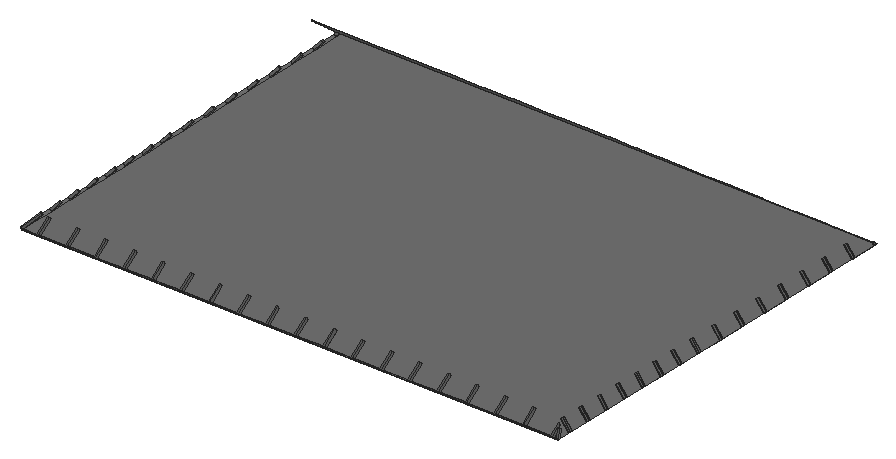
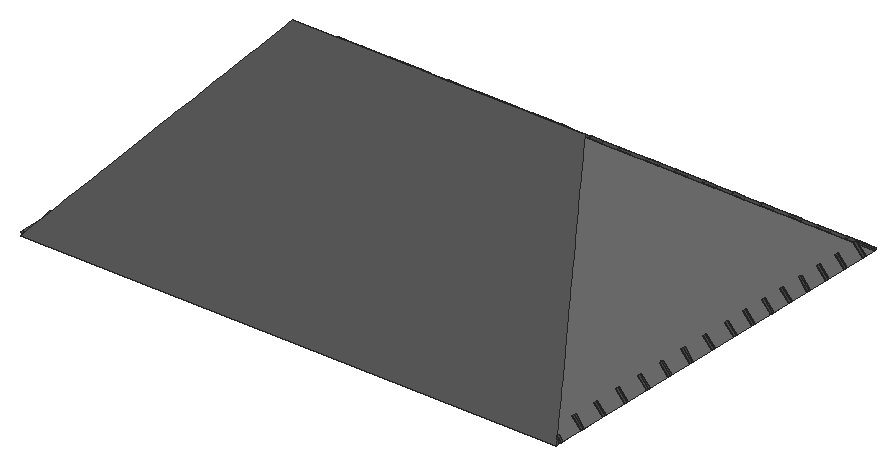
# SketchUp Ruby script. Lengths in inches.
U = 1.inch
M = Sketchup.active_model
def pt(a) = Geom::Point3d.new(a.map { |v| v * U })
def face(e, loops, mat)
  f = e.add_face(loops[0].map { |a| pt(a) })
  loops[1..].each { |l| e.add_face(l.map { |a| pt(a) }).erase! }
  f.material = f.back_material = mat if mat
  f
end
# faces: each face lists its corners as indices into pts; further lists are holes
def faces(e, pts, list, mat = nil) = list.each { |f| face(e, (f[0].is_a?(Array) ? f : [f]).map { |l| l.map { |i| pts[i] } }, mat) }
# xy, xz, yz: faces in a plane at the given z, y or x. An outline is a flat list of corners, or four numbers for a rectangle; further outlines are holes
def ring(l) = l.size == 4 ? [[l[0], l[1]], [l[2], l[1]], [l[2], l[3]], [l[0], l[3]]] : l.each_slice(2).to_a
def flat(e, list, mat, &to3) = list.each { |f| face(e, (f[0].is_a?(Array) ? f : [f]).map { |l| ring(l).map { |u, v| to3.(u, v) } }, mat) }
def xy(e, z, list, mat = nil) = flat(e, list, mat) { |x, y| [x, y, z] }
def xz(e, y, list, mat = nil) = flat(e, list, mat) { |x, z| [x, y, z] }
def yz(e, x, list, mat = nil) = flat(e, list, mat) { |y, z| [x, y, z] }
def lines(e, pts, list) = list.each { |a, b| e.add_line(pt(pts[a]), pt(pts[b])) }
# prism: a flat outline (further loops are holes) pulled along v
def prism(e, loops, v, mat = nil)
  f = face(e, loops, mat); d = Geom::Vector3d.new(v.map { |x| x * U })
  f.pushpull(f.normal.samedirection?(d) ? d.length : -d.length)
end
def box(e, o, s, mat = nil) = prism(e, [[o, [o[0] + s[0], o[1], o[2]], [o[0] + s[0], o[1] + s[1], o[2]], [o[0], o[1] + s[1], o[2]]]], [0, 0, s[2]], mat)
def at(x, y, z, deg = 0) = Geom::Transformation.translation(pt([x, y, z])) * Geom::Transformation.rotation(ORIGIN, Z_AXIS, deg.degrees)
def axes(o, x, y, z) = Geom::Transformation.new([*x, 0, *y, 0, *z, 0, *pt(o).to_a, 1])
def part(name) = M.definitions.add(name)
# library, detail: a bought-in or finely detailed component or shape, given as its bounding box
def library(name, o, s) = part(name).tap { |d| box(d.entities, o, s) }
def detail(e, o, s) = box(e.add_group.entities, o, s)
def put(e, d, t, mat = nil) = e.add_instance(d, t).tap { |i| i.material = mat if mat }
def group(e, t, mat = nil) = e.add_group.tap { |g| g.transformation = t; g.material = mat if mat }.entities
root = M.entities
M.materials.add("[Color M05]").color = [114, 114, 114]
xy(root,407.09,[[338.37,286.64,788.76,621.71]],"[Color M05]")
xz(root,298,[[338.37,407.09,336.88,408.43,344.33,416.75,345.82,415.41],[788.76,407.09,782.3,415.41,783.88,416.64,790.34,408.32]],"[Color M05]")
xz(root,299.21,[[338.37,407.09,345.82,415.41,344.33,416.75,336.88,408.43],[788.76,407.09,790.34,408.32,783.88,416.64,782.3,415.41]],"[Color M05]")
xz(root,317.375,[[338.37,407.09,336.88,408.43,344.33,416.75,345.82,415.41],[788.76,407.09,782.3,415.41,783.88,416.64,790.34,408.32]],"[Color M05]")
xz(root,318.58,[[338.37,407.09,345.82,415.41,344.33,416.75,336.88,408.43],[788.76,407.09,790.34,408.32,783.88,416.64,782.3,415.41]],"[Color M05]")
xz(root,336.74,[[338.37,407.09,336.88,408.43,344.33,416.75,345.82,415.41],[788.76,407.09,782.3,415.41,783.88,416.64,790.34,408.32]],"[Color M05]")
xz(root,337.95,[[338.37,407.09,345.82,415.41,344.33,416.75,336.88,408.43],[788.76,407.09,790.34,408.32,783.88,416.64,782.3,415.41]],"[Color M05]")
xz(root,356.11,[[338.37,407.09,336.88,408.43,344.33,416.75,345.82,415.41],[788.76,407.09,782.3,415.41,783.88,416.64,790.34,408.32]],"[Color M05]")
xz(root,357.32,[[338.37,407.09,345.82,415.41,344.33,416.75,336.88,408.43],[788.76,407.09,790.34,408.32,783.88,416.64,782.3,415.41]],"[Color M05]")
xz(root,375.48,[[338.37,407.09,336.88,408.43,344.33,416.75,345.82,415.41],[788.76,407.09,782.3,415.41,783.88,416.64,790.34,408.32]],"[Color M05]")
xz(root,376.69,[[338.37,407.09,345.82,415.41,344.33,416.75,336.88,408.43],[788.76,407.09,790.34,408.32,783.88,416.64,782.3,415.41]],"[Color M05]")
xz(root,394.85,[[338.37,407.09,336.88,408.43,344.33,416.75,345.82,415.41],[788.76,407.09,782.3,415.41,783.88,416.64,790.34,408.32]],"[Color M05]")
xz(root,396.0625,[[338.37,407.09,345.82,415.41,344.33,416.75,336.88,408.43],[788.76,407.09,790.34,408.32,783.88,416.64,782.3,415.41]],"[Color M05]")
xz(root,414.22,[[338.37,407.09,336.88,408.43,344.33,416.75,345.82,415.41],[788.76,407.09,782.3,415.41,783.88,416.64,790.34,408.32]],"[Color M05]")
xz(root,415.43,[[338.37,407.09,345.82,415.41,344.33,416.75,336.88,408.43],[788.76,407.09,790.34,408.32,783.88,416.64,782.3,415.41]],"[Color M05]")
xz(root,433.3,[[338.37,407.09,336.88,408.43,344.33,416.75,345.82,415.41]],"[Color M05]")
xz(root,433.59,[[788.76,407.09,782.3,415.41,783.88,416.64,790.34,408.32]],"[Color M05]")
xz(root,434.8,[[338.37,407.09,345.82,415.41,344.33,416.75,336.88,408.43],[788.76,407.09,790.34,408.32,783.88,416.64,782.3,415.41]],"[Color M05]")
xz(root,456.21,[[338.37,407.09,336.88,408.43,344.33,416.75,345.82,415.41]],"[Color M05]")
xz(root,456.8,[[788.76,407.09,782.3,415.41,783.88,416.64,790.34,408.32]],"[Color M05]")
xz(root,457.71,[[338.37,407.09,345.82,415.41,344.33,416.75,336.88,408.43]],"[Color M05]")
xz(root,458.01,[[788.76,407.09,790.34,408.32,783.88,416.64,782.3,415.41]],"[Color M05]")
xz(root,479.13,[[338.37,407.09,336.88,408.43,344.33,416.75,345.82,415.41]],"[Color M05]")
xz(root,480.02,[[788.76,407.09,782.3,415.41,783.88,416.64,790.34,408.32]],"[Color M05]")
xz(root,480.63,[[338.37,407.09,345.82,415.41,344.33,416.75,336.88,408.43]],"[Color M05]")
xz(root,481.23,[[788.76,407.09,790.34,408.32,783.88,416.64,782.3,415.41]],"[Color M05]")
xz(root,502.04,[[338.37,407.09,336.88,408.43,344.33,416.75,345.82,415.41]],"[Color M05]")
xz(root,503.23,[[788.76,407.09,782.3,415.41,783.88,416.64,790.34,408.32]],"[Color M05]")
xz(root,503.54,[[338.37,407.09,345.82,415.41,344.33,416.75,336.88,408.43]],"[Color M05]")
xz(root,504.44,[[788.76,407.09,790.34,408.32,783.88,416.64,782.3,415.41]],"[Color M05]")
xz(root,524.95,[[338.37,407.09,336.88,408.43,344.33,416.75,345.82,415.41]],"[Color M05]")
xz(root,526.45,[[338.37,407.09,345.82,415.41,344.33,416.75,336.88,408.43],[788.76,407.09,782.3,415.41,783.88,416.64,790.34,408.32]],"[Color M05]")
xz(root,527.66,[[788.76,407.09,790.34,408.32,783.88,416.64,782.3,415.41]],"[Color M05]")
xz(root,547.87,[[338.37,407.09,336.88,408.43,344.33,416.75,345.82,415.41]],"[Color M05]")
xz(root,549.37,[[338.37,407.09,345.82,415.41,344.33,416.75,336.88,408.43]],"[Color M05]")
xz(root,549.66,[[788.76,407.09,782.3,415.41,783.88,416.64,790.34,408.32]],"[Color M05]")
xz(root,550.87,[[788.76,407.09,790.34,408.32,783.88,416.64,782.3,415.41]],"[Color M05]")
xz(root,570.78,[[338.37,407.09,336.88,408.43,344.33,416.75,345.82,415.41]],"[Color M05]")
xz(root,572.28,[[338.37,407.09,345.82,415.41,344.33,416.75,336.88,408.43]],"[Color M05]")
xz(root,572.875,[[788.76,407.09,782.3,415.41,783.88,416.64,790.34,408.32]],"[Color M05]")
xz(root,574.08,[[788.76,407.09,790.34,408.32,783.88,416.64,782.3,415.41]],"[Color M05]")
xz(root,593.69,[[338.37,407.09,336.88,408.43,344.33,416.75,345.82,415.41]],"[Color M05]")
xz(root,595.19,[[338.37,407.09,345.82,415.41,344.33,416.75,336.88,408.43]],"[Color M05]")
xz(root,596.09,[[788.76,407.09,782.3,415.41,783.88,416.64,790.34,408.32]],"[Color M05]")
xz(root,597.3,[[788.76,407.09,790.34,408.32,783.88,416.64,782.3,415.41]],"[Color M05]")
xz(root,616.61,[[338.37,407.09,336.88,408.43,340.22,412.16,341.71,410.82]],"[Color M05]")
xz(root,618.11,[[338.37,407.09,340.73,409.73,339.24,411.06,336.88,408.43]],"[Color M05]")
xz(root,619.3,[[788.76,407.09,787.4,408.85,788.98,410.08,790.34,408.32]],"[Color M05]")
yz(root,352.12,[[286.64,407.09,298,415.41,296.82,417.03,285.45,408.71]],"[Color M05]")
yz(root,353.62,[[286.64,407.09,285.45,408.71,296.82,417.03,298,415.41]],"[Color M05]")
yz(root,376.12,[[286.64,407.09,298,415.41,296.82,417.03,285.45,408.71]],"[Color M05]")
yz(root,377.62,[[286.64,407.09,285.45,408.71,296.82,417.03,298,415.41]],"[Color M05]")
yz(root,400.12,[[286.64,407.09,298,415.41,296.82,417.03,285.45,408.71]],"[Color M05]")
yz(root,401.62,[[286.64,407.09,285.45,408.71,296.82,417.03,298,415.41]],"[Color M05]")
yz(root,424.12,[[286.64,407.09,298,415.41,296.82,417.03,285.45,408.71]],"[Color M05]")
yz(root,425.62,[[286.64,407.09,285.45,408.71,296.82,417.03,298,415.41]],"[Color M05]")
yz(root,448.12,[[286.64,407.09,298,415.41,296.82,417.03,285.45,408.71]],"[Color M05]")
yz(root,449.62,[[286.64,407.09,285.45,408.71,296.82,417.03,298,415.41]],"[Color M05]")
yz(root,472.12,[[286.64,407.09,298,415.41,296.82,417.03,285.45,408.71]],"[Color M05]")
yz(root,473.62,[[286.64,407.09,285.45,408.71,296.82,417.03,298,415.41]],"[Color M05]")
yz(root,496.12,[[286.64,407.09,298,415.41,296.82,417.03,285.45,408.71]],"[Color M05]")
yz(root,497.62,[[286.64,407.09,285.45,408.71,296.82,417.03,298,415.41]],"[Color M05]")
yz(root,520.12,[[286.64,407.09,298,415.41,296.82,417.03,285.45,408.71]],"[Color M05]")
yz(root,521.62,[[286.64,407.09,285.45,408.71,296.82,417.03,298,415.41]],"[Color M05]")
yz(root,544.12,[[286.64,407.09,298,415.41,296.82,417.03,285.45,408.71]],"[Color M05]")
yz(root,545.62,[[286.64,407.09,285.45,408.71,296.82,417.03,298,415.41]],"[Color M05]")
yz(root,568.12,[[286.64,407.09,298,415.41,296.82,417.03,285.45,408.71]],"[Color M05]")
yz(root,569.62,[[286.64,407.09,285.45,408.71,296.82,417.03,298,415.41]],"[Color M05]")
yz(root,592.12,[[286.64,407.09,298,415.41,296.82,417.03,285.45,408.71]],"[Color M05]")
yz(root,593.62,[[286.64,407.09,285.45,408.71,296.82,417.03,298,415.41]],"[Color M05]")
yz(root,616.15,[[286.64,407.09,298,415.41,296.82,417.03,285.45,408.71]],"[Color M05]")
yz(root,617.62,[[286.64,407.09,285.45,408.71,296.82,417.03,298,415.41]],"[Color M05]")
yz(root,640.12,[[286.64,407.09,298,415.41,296.82,417.03,285.45,408.71]],"[Color M05]")
yz(root,641.62,[[286.64,407.09,285.45,408.71,296.82,417.03,298,415.41]],"[Color M05]")
yz(root,664.12,[[286.64,407.09,298,415.41,296.82,417.03,285.45,408.71]],"[Color M05]")
yz(root,665.62,[[286.64,407.09,285.45,408.71,296.82,417.03,298,415.41]],"[Color M05]")
yz(root,688.12,[[286.64,407.09,298,415.41,296.82,417.03,285.45,408.71]],"[Color M05]")
yz(root,689.62,[[286.64,407.09,285.45,408.71,296.82,417.03,298,415.41]],"[Color M05]")
yz(root,712.12,[[286.64,407.09,298,415.41,296.82,417.03,285.45,408.71]],"[Color M05]")
yz(root,713.62,[[286.64,407.09,285.45,408.71,296.82,417.03,298,415.41]],"[Color M05]")
yz(root,736.12,[[286.64,407.09,298,415.41,296.82,417.03,285.45,408.71]],"[Color M05]")
yz(root,737.62,[[286.64,407.09,285.45,408.71,296.82,417.03,298,415.41]],"[Color M05]")
yz(root,760.12,[[286.64,407.09,298,415.41,296.82,417.03,285.45,408.71]],"[Color M05]")
yz(root,761.62,[[286.64,407.09,285.45,408.71,296.82,417.03,298,415.41]],"[Color M05]")
yz(root,784.12,[[286.64,407.09,294.8,413.07,293.62,414.68,285.45,408.71]],"[Color M05]")
yz(root,785.62,[[286.64,407.09,285.45,408.71,290.98,412.75,292.16,411.14]],"[Color M05]")
p = [[338.37,286.64,407.09],[352.12,286.64,407.09],[352.12,285.45,408.71],[338.37,285.45,408.71],[345.82,298,415.41],[345.82,296.82,417.03],
  [353.62,286.64,407.09],[376.12,286.64,407.09],[376.12,285.45,408.71],[353.62,285.45,408.71],[377.62,286.64,407.09],[400.12,286.64,407.09],
  [400.12,285.45,408.71],[377.62,285.45,408.71],[401.62,286.64,407.09],[424.12,286.64,407.09],[424.12,285.45,408.71],[401.62,285.45,408.71],
  [425.62,286.64,407.09],[448.12,286.64,407.09],[448.12,285.45,408.71],[425.62,285.45,408.71],[449.62,286.64,407.09],[472.12,286.64,407.09],
  [472.12,285.45,408.71],[449.62,285.45,408.71],[473.62,286.64,407.09],[496.12,286.64,407.09],[496.12,285.45,408.71],[473.62,285.45,408.71],
  [497.62,286.64,407.09],[520.12,286.64,407.09],[520.12,285.45,408.71],[497.62,285.45,408.71],[521.62,286.64,407.09],[544.12,286.64,407.09],
  [544.12,285.45,408.71],[521.62,285.45,408.71],[545.62,286.64,407.09],[568.12,286.64,407.09],[568.12,285.45,408.71],[545.62,285.45,408.71],
  [569.62,286.64,407.09],[592.12,286.64,407.09],[592.12,285.45,408.71],[569.62,285.45,408.71],[593.62,286.64,407.09],[616.15,286.64,407.09],
  [616.15,285.45,408.71],[593.62,285.45,408.71],[617.62,286.64,407.09],[640.12,286.64,407.09],[640.12,285.45,408.71],[617.62,285.45,408.71],
  [641.62,286.64,407.09],[664.12,286.64,407.09],[664.12,285.45,408.71],[641.62,285.45,408.71],[665.62,286.64,407.09],[688.12,286.64,407.09],
  [688.12,285.45,408.71],[665.62,285.45,408.71],[689.62,286.64,407.09],[712.12,286.64,407.09],[712.12,285.45,408.71],[689.62,285.45,408.71],
  [713.62,286.64,407.09],[736.12,286.64,407.09],[736.12,285.45,408.71],[713.62,285.45,408.71],[737.62,286.64,407.09],[760.12,286.64,407.09],
  [760.12,285.45,408.71],[737.62,285.45,408.71],[761.62,286.64,407.09],[784.12,286.64,407.09],[784.12,285.45,408.71],[761.62,285.45,408.71],
  [788.76,286.64,407.09],[785.62,292.16,411.14],[785.62,290.98,412.75],[788.76,285.45,408.71],[785.62,286.64,407.09],[785.62,285.45,408.71],
  [344.33,298,416.75],[336.88,286.64,408.43],[338.37,298,407.09],[336.88,298,408.43],[353.62,298,415.41],[352.12,298,415.41],
  [377.62,298,415.41],[376.12,298,415.41],[401.62,298,415.41],[400.12,298,415.41],[425.62,298,415.41],[424.12,298,415.41],
  [449.62,298,415.41],[448.12,298,415.41],[473.62,298,415.41],[472.12,298,415.41],[497.62,298,415.41],[496.12,298,415.41],
  [521.62,298,415.41],[520.12,298,415.41],[545.62,298,415.41],[544.12,298,415.41],[569.62,298,415.41],[568.12,298,415.41],
  [593.62,298,415.41],[592.12,298,415.41],[617.62,298,415.41],[616.15,298,415.41],[641.62,298,415.41],[640.12,298,415.41],
  [665.62,298,415.41],[664.12,298,415.41],[689.62,298,415.41],[688.12,298,415.41],[713.62,298,415.41],[712.12,298,415.41],
  [737.62,298,415.41],[736.12,298,415.41],[761.62,298,415.41],[760.12,298,415.41],[784.12,294.8,413.07],[790.34,286.64,408.32],
  [787.2,292.16,412.36],[788.76,298,407.09],[790.34,298,408.32],[345.82,299.21,415.41],[338.37,299.21,407.09],[788.76,299.21,407.09],
  [782.3,299.21,415.41],[782.3,298,415.41],[338.37,317.375,407.09],[336.88,299.21,408.43],[336.88,317.375,408.43],[788.76,317.375,407.09],
  [790.34,317.375,408.32],[790.34,299.21,408.32],[338.37,318.58,407.09],[345.82,317.375,415.41],[345.82,318.58,415.41],[788.76,318.58,407.09],
  [782.3,318.58,415.41],[782.3,317.375,415.41],[338.37,336.74,407.09],[336.88,318.58,408.43],[336.88,336.74,408.43],[788.76,336.74,407.09],
  [790.34,336.74,408.32],[790.34,318.58,408.32],[338.37,337.95,407.09],[345.82,336.74,415.41],[345.82,337.95,415.41],[788.76,337.95,407.09],
  [782.3,337.95,415.41],[782.3,336.74,415.41],[338.37,356.11,407.09],[336.88,337.95,408.43],[336.88,356.11,408.43],[788.76,356.11,407.09],
  [790.34,356.11,408.32],[790.34,337.95,408.32],[338.37,357.32,407.09],[345.82,356.11,415.41],[345.82,357.32,415.41],[788.76,357.32,407.09],
  [782.3,357.32,415.41],[782.3,356.11,415.41],[338.37,375.48,407.09],[336.88,357.32,408.43],[336.88,375.48,408.43],[788.76,375.48,407.09],
  [790.34,375.48,408.32],[790.34,357.32,408.32],[345.82,375.48,415.41],[345.82,376.69,415.41],[338.37,376.69,407.09],[788.76,376.69,407.09],
  [782.3,376.69,415.41],[782.3,375.48,415.41],[338.37,394.85,407.09],[336.88,376.69,408.43],[336.88,394.85,408.43],[788.76,394.85,407.09],
  [790.34,394.85,408.32],[790.34,376.69,408.32],[338.37,396.0625,407.09],[345.82,394.85,415.41],[345.82,396.0625,415.41],[788.76,396.0625,407.09],
  [782.3,396.0625,415.41],[782.3,394.85,415.41],[338.37,414.22,407.09],[336.88,396.0625,408.43],[336.88,414.22,408.43],[788.76,414.22,407.09],
  [790.34,414.22,408.32],[790.34,396.0625,408.32],[338.37,415.43,407.09],[345.82,414.22,415.41],[345.82,415.43,415.41],[788.76,415.43,407.09],
  [782.3,415.43,415.41],[782.3,414.22,415.41],[338.37,433.3,407.09],[336.88,415.43,408.43],[336.88,433.3,408.43],[788.76,433.59,407.09],
  [790.34,433.59,408.32],[790.34,415.43,408.32],[338.37,434.8,407.09],[345.82,433.3,415.41],[345.82,434.8,415.41],[788.76,434.8,407.09],
  [782.3,434.8,415.41],[782.3,433.59,415.41],[338.37,456.21,407.09],[336.88,434.8,408.43],[336.88,456.21,408.43],[788.76,456.8,407.09],
  [790.34,456.8,408.32],[790.34,434.8,408.32],[448.12,454.17,529.67],[449.62,454.17,529.67],[472.12,454.17,529.67],[473.62,454.17,529.67],
  [496.12,454.17,529.67],[497.62,454.17,529.67],[520.12,454.17,529.67],[521.62,454.17,529.67],[544.12,454.17,529.67],[545.62,454.17,529.67],
  [568.12,454.17,529.67],[569.62,454.17,529.67],[592.12,454.17,529.67],[593.62,454.17,529.67],[616.12,454.17,529.67],[617.62,454.17,529.67],
  [640.12,454.17,529.67],[641.62,454.17,529.67],[664.12,454.17,529.67],[665.62,454.17,529.67],[688.12,454.17,529.67],[689.62,454.17,529.67],
  [693.5625,454.17,529.67],[695.0625,456.8,527.74],[695.75,458.01,526.85],[704.57,473.54,515.5],[705.26,474.75,514.61],[708.25,480.02,510.76],
  [708.94,481.23,509.87],[715.58,492.91,501.32],[716.26,494.12,500.4375],[721.44,503.23,493.77],[722.13,504.44,492.89],[726.58,512.28,487.15],
  [727.27,513.49,486.27],[734.63,526.45,476.79],[735.32,527.66,475.9],[737.59,531.65,472.98],[738.28,532.86,472.1],[747.82,549.66,459.8],
  [748.5,550.86,458.93],[748.6,551.02,458.81],[749.28,552.23,457.92],[759.6,570.39,444.64],[760.29,571.6,443.75],[761.02,572.875,442.82],
  [761.7,574.08,441.93],[770.61,589.76,430.47],[771.3,590.97,429.58],[774.21,596.09,425.84],[774.89,597.3,424.95],[781.61,609.125,416.3],
  [782.3,610.34,415.41],[787.4,619.3,408.85],[788.09,620.51,407.97],[788.76,621.71,407.09],[338.37,621.71,407.09],[340.73,618.11,409.73],
  [341.71,616.61,410.82],[345.82,610.34,415.41],[346.61,609.125,416.3],[355.74,595.19,426.49],[356.72,593.69,427.59],[358.51,590.97,429.58],
  [359.3,589.76,430.47],[370.75,572.28,443.25],[371.2,571.6,443.75],[371.73,570.78,444.35],[371.99,570.39,444.64],[383.89,552.23,457.92],
  [384.68,551.02,458.81],[385.76,549.37,460.02],[386.74,547.87,461.11],[396.57,532.86,472.1],[397.37,531.65,472.98],[400.77,526.45,476.78],
  [401.75,524.95,477.88],[409.26,513.49,486.27],[410.06,512.28,487.15],[415.78,503.54,493.55],[416.76,502.04,494.64],[421.95,494.12,500.4375],
  [422.75,492.91,501.32],[430.79,480.63,510.31],[431.77,479.13,511.41],[434.64,474.75,514.61],[435.43,473.54,515.5],[445.8,457.71,527.07],
  [446.78,456.21,528.17],[338.37,457.71,407.09],[345.82,456.21,415.41],[345.82,457.71,415.41],[788.76,458.01,407.09],[782.3,458.01,415.41],
  [782.3,456.8,415.41],[338.37,479.13,407.09],[336.88,457.71,408.43],[336.88,479.13,408.43],[788.76,480.02,407.09],[790.34,480.02,408.32],
  [790.34,458.01,408.32],[338.37,480.63,407.09],[345.82,479.13,415.41],[345.82,480.63,415.41],[788.76,481.23,407.09],[782.3,481.23,415.41],
  [782.3,480.02,415.41],[338.37,502.04,407.09],[336.88,480.63,408.43],[336.88,502.04,408.43],[788.76,503.23,407.09],[790.34,503.23,408.32],
  [790.34,481.23,408.32],[338.37,503.54,407.09],[345.82,502.04,415.41],[345.82,503.54,415.41],[788.76,504.44,407.09],[782.3,504.44,415.41],
  [782.3,503.23,415.41],[338.37,524.95,407.09],[336.88,503.54,408.43],[336.88,524.95,408.43],[788.76,526.45,407.09],[790.34,526.45,408.32],
  [790.34,504.44,408.32],[338.37,526.45,407.09],[345.82,524.95,415.41],[345.82,526.45,415.41],[788.76,527.66,407.09],[782.3,527.66,415.41],
  [782.3,526.45,415.41],[338.37,547.87,407.09],[336.88,526.45,408.43],[336.88,547.87,408.43],[788.76,549.66,407.09],[790.34,549.66,408.32],
  [790.34,527.66,408.32],[338.37,549.37,407.09],[345.82,547.87,415.41],[345.82,549.37,415.41],[338.37,570.78,407.09],[336.88,549.37,408.43],
  [336.88,570.78,408.43],[788.76,550.87,407.09],[782.3,550.87,415.41],[782.3,549.66,415.41],[788.76,572.875,407.09],[790.34,572.875,408.32],
  [790.34,550.87,408.32],[338.37,572.28,407.09],[345.82,570.78,415.41],[345.82,572.28,415.41],[338.37,593.69,407.09],[336.88,572.28,408.43],
  [336.88,593.69,408.43],[788.76,574.08,407.09],[782.3,574.08,415.41],[782.3,572.875,415.41],[788.76,596.09,407.09],[790.34,596.09,408.32],
  [790.34,574.08,408.32],[338.37,595.19,407.09],[345.82,593.69,415.41],[345.82,595.19,415.41],[338.37,616.61,407.09],[336.88,595.19,408.43],
  [336.88,616.61,408.43],[788.76,597.3,407.09],[782.3,597.3,415.41],[782.3,596.09,415.41],[788.76,619.3,407.09],[790.34,619.3,408.32],
  [790.34,597.3,408.32],[338.37,618.11,407.09],[336.88,618.11,408.43],[336.88,621.71,408.43],[339.24,618.11,411.06],[788.76,620.51,407.09]]
faces(root,p,[[0,1,2,3],[4,0,3,5],[6,7,8,9],[10,11,12,13],[14,15,16,17],[18,19,20,21],[22,23,24,25],[26,27,28,29],
  [30,31,32,33],[34,35,36,37],[38,39,40,41],[42,43,44,45],[46,47,48,49],[50,51,52,53],[54,55,56,57],[58,59,60,61],
  [62,63,64,65],[66,67,68,69],[70,71,72,73],[74,75,76,77],[78,79,80,81],[82,78,81,83],[0,4,84,85],[86,0,85,87],
  [1,6,88,89],[7,10,90,91],[11,14,92,93],[15,18,94,95],[19,22,96,97],[23,26,98,99],[27,30,100,101],[31,34,102,103],
  [35,38,104,105],[39,42,106,107],[43,46,108,109],[47,50,110,111],[51,54,112,113],[55,58,114,115],[59,62,116,117],[63,66,118,119],
  [67,70,120,121],[71,74,122,123],[79,124,75,82],[79,78,125,126],[78,127,128,125],[4,129,130,86],[131,132,133,127],[134,130,135,136],
  [131,137,138,139],[140,134,141,142],[137,143,144,145],[146,140,147,148],[143,149,150,151],[152,146,153,154],[149,155,156,157],[158,152,159,160],
  [155,161,162,163],[164,158,165,166],[161,167,168,169],[170,164,171,172],[167,173,174,175],[176,177,178,170],[173,179,180,181],[182,178,183,184],
  [179,185,186,187],[188,182,189,190],[185,191,192,193],[194,188,195,196],[191,197,198,199],[200,194,201,202],[197,203,204,205],[206,200,207,208],
  [203,209,210,211],[212,206,213,214],[209,215,216,217],[218,212,219,220],[215,221,222,223],[224,225,226,227,228,229,230,231,232,233,234,235,236,237,238,239,240,241,242,243,244,245,246,247,248,249,250,251,252,253,254,255,256,257,258,259,260,261,262,263,264,265,266,267,268,269,270,271,272,273,274,275,276,277,278,279,280,281,282,283,284,285,286,287,288,289,290,291,292,293,294,295,296,297,298,299,300,301,302,303,304,305,306,307,308,309,310,311,312],[313,218,314,315],[221,316,317,318],
  [319,313,320,321],[316,322,323,324],[325,319,326,327],[322,328,329,330],[331,325,332,333],[328,334,335,336],[337,331,338,339],[334,340,341,342],
  [343,337,344,345],[340,346,347,348],[349,343,350,351],[346,352,353,354],[355,349,356,357],[352,358,359,360],[361,355,362,363],[364,361,365,366],
  [358,367,368,369],[367,370,371,372],[373,364,374,375],[376,373,377,378],[370,379,380,381],[379,382,383,384],[385,376,386,387],[388,385,389,390],
  [382,391,392,393],[391,394,395,396],[397,388,282,281],[280,397,398,399],[281,280,399,400],[278,277,394,401],[279,278,401]],"[Color M05]")
